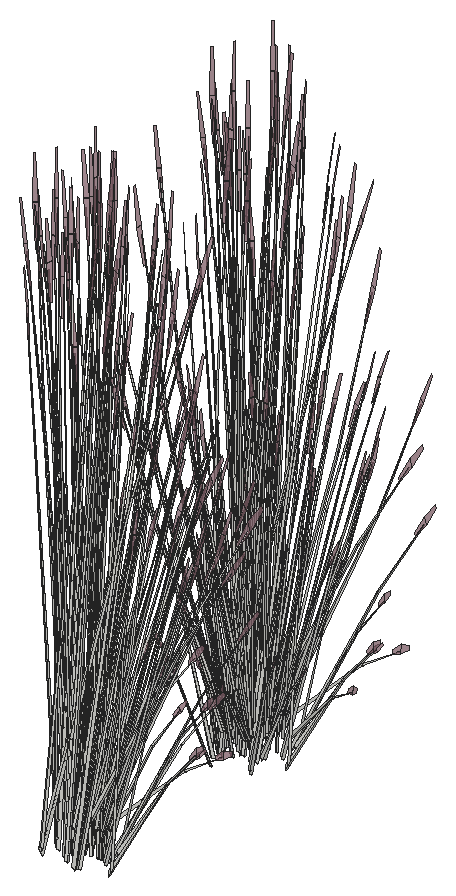
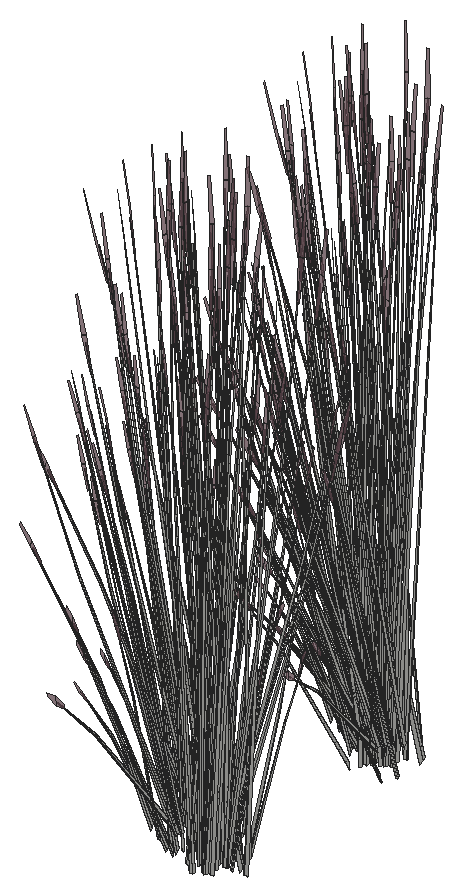
# SketchUp Ruby script. Lengths in inches.
U = 1.inch
M = Sketchup.active_model
def pt(a) = Geom::Point3d.new(a.map { |v| v * U })
def face(e, loops, mat)
  f = e.add_face(loops[0].map { |a| pt(a) })
  loops[1..].each { |l| e.add_face(l.map { |a| pt(a) }).erase! }
  f.material = f.back_material = mat if mat
  f
end
# faces: each face lists its corners as indices into pts; further lists are holes
def faces(e, pts, list, mat = nil) = list.each { |f| face(e, (f[0].is_a?(Array) ? f : [f]).map { |l| l.map { |i| pts[i] } }, mat) }
# xy, xz, yz: faces in a plane at the given z, y or x. An outline is a flat list of corners, or four numbers for a rectangle; further outlines are holes
def ring(l) = l.size == 4 ? [[l[0], l[1]], [l[2], l[1]], [l[2], l[3]], [l[0], l[3]]] : l.each_slice(2).to_a
def flat(e, list, mat, &to3) = list.each { |f| face(e, (f[0].is_a?(Array) ? f : [f]).map { |l| ring(l).map { |u, v| to3.(u, v) } }, mat) }
def xy(e, z, list, mat = nil) = flat(e, list, mat) { |x, y| [x, y, z] }
def xz(e, y, list, mat = nil) = flat(e, list, mat) { |x, z| [x, y, z] }
def yz(e, x, list, mat = nil) = flat(e, list, mat) { |y, z| [x, y, z] }
def lines(e, pts, list) = list.each { |a, b| e.add_line(pt(pts[a]), pt(pts[b])) }
# prism: a flat outline (further loops are holes) pulled along v
def prism(e, loops, v, mat = nil)
  f = face(e, loops, mat); d = Geom::Vector3d.new(v.map { |x| x * U })
  f.pushpull(f.normal.samedirection?(d) ? d.length : -d.length)
end
def box(e, o, s, mat = nil) = prism(e, [[o, [o[0] + s[0], o[1], o[2]], [o[0] + s[0], o[1] + s[1], o[2]], [o[0], o[1] + s[1], o[2]]]], [0, 0, s[2]], mat)
def at(x, y, z, deg = 0) = Geom::Transformation.translation(pt([x, y, z])) * Geom::Transformation.rotation(ORIGIN, Z_AXIS, deg.degrees)
def axes(o, x, y, z) = Geom::Transformation.new([*x, 0, *y, 0, *z, 0, *pt(o).to_a, 1])
def part(name) = M.definitions.add(name)
# library, detail: a bought-in or finely detailed component or shape, given as its bounding box
def library(name, o, s) = part(name).tap { |d| box(d.entities, o, s) }
def detail(e, o, s) = box(e.add_group.entities, o, s)
def put(e, d, t, mat = nil) = e.add_instance(d, t).tap { |i| i.material = mat if mat }
def group(e, t, mat = nil) = e.add_group.tap { |g| g.transformation = t; g.material = mat if mat }.entities
root = M.entities
M.materials.add("LightPink_Translucent").color = [144, 107, 117]
M.materials["LightPink_Translucent"].alpha = 0.75
c1 = part("blade")
p = [[2.15,0.21,22],[0,0.17,0],[0.09,0.45,0],[2.18,0.31,22],[2.29,0.31,22],[0.38,0.45,0],
  [2.48,0.24,33],[2.49,0.24,33],[2.48,0.22,33]]
faces(c1.entities,p,[[0,1,2,3],[4,5,2,3],[6,3,4,7],[8,0,3,6]])
c2 = part("seeds")
p = [[0.3,-0.1,1.38],[-0.01,-0.03,1.59],[-0.01,-0.03,0.03],[0.14,-0.07,-0.07],[0.29,-0.03,3],[0.15,0.01,3.11]]
faces(c2.entities,p,[[0,1,2,3],[1,0,4,5]],"LightPink_Translucent")
c3 = part("blade with seeds")
put(c3.entities,c1,at(0,0,0))
put(c3.entities,c2,axes([2.4,0.25,30.99],[1.5799,-0.05474,1.17369],[-0.12525,1.92788,0.29478],[-0.07173,-0.02425,1.56792]))
put(root,c3,axes([509.35,499.15,3.875],[0.20584,-0.55581,-0.51099],[0.70573,0.19051,-0.3958],[0.28414,-0.05097,0.97773]))
put(root,c3,axes([508.24,496.89,1.57],[0.47504,-0.61229,0],[0.79476,0.34146,-0.51607],[0.18101,0.07777,1.63711]))
put(root,c3,axes([505.49,498.78,1.55],[0.33034,0.68327,0.45755],[-0.94388,0.2376,0.17955],[0.01154,-0.12555,1.58856]))
put(root,c3,axes([510.11,499.31,1.17],[-0.48937,0.07333,1.41583],[-0.07789,-0.58369,0.08104],[0.34275,-0.08835,0.80566]))
put(root,c3,axes([511,498.79,1.45],[-0.47106,-0.39072,-0.06488],[0.51591,-0.35801,-0.29416],[0.14618,-0.02521,0.97024]))
put(root,c3,axes([505.32,499.32,1.91],[-0.36864,0.55059,0.44739],[-0.76598,-0.26498,-0.21531],[0,-0.12692,1.43643]))
put(root,c3,axes([506.67,498.84,1.4],[0,-0.70701,0],[0.95008,0,0],[0,0,1.79456]))
put(root,c3,axes([507.83,497.21,1.67],[-0.7111,-0.30552,0.49651],[0.42504,-0.54784,0],[0.16196,0.06958,1.57504]))
put(root,c3,axes([509.22,499.35,4.17],[0.66765,-0.26986,-0.71045],[0.37208,0.55551,0.08574],[0.32259,-0.0631,1.00501]))
put(root,c3,axes([506.22,498.39,1.55],[-0.62999,0.55453,0.45755],[-0.74845,-0.4895,0.17955],[0.15188,-0.05534,1.58856]))
put(root,c3,axes([506.91,499.39,1.49],[-0.70674,-0.52593,-0.06131],[0.70717,-0.52625,0],[-0.02468,-0.01837,1.75571]))
put(root,c3,axes([505.13,497.48,1.67],[-0.21949,0.60727,0.17642],[-0.8032,-0.17185,0.35086],[0.13875,-0.00296,1.60407]))
put(root,c3,axes([509.12,499.46,4.24],[-0.63144,-0.17046,0.35414],[0.18417,-0.49731,-0.4572],[0.25423,-0.0456,0.87481]))
put(root,c3,axes([504.8,497.97,0.79],[-0.74787,0.24464,1.28929],[-0.23804,-0.70192,0.50096],[0.45924,0.01168,1.46642]))
put(root,c3,axes([506.81,498.16,1.81],[0.14658,-0.54532,0.1448],[0.71613,0.09466,-0.41347],[0.13033,0.05599,1.26744]))
put(root,c3,axes([505.57,499.45,1.55],[0.96033,0.12874,0.45755],[-0.19544,0.7271,0.17955],[-0.14034,-0.07021,1.58856]))
put(root,c3,axes([510.64,498.92,0.6875],[-0.03971,-0.09277,1.76342],[0.27541,-0.54264,-0.26939],[0.27782,-0.00781,0.30037]))
put(root,c3,axes([506.5,498.3,1.91],[-0.45644,-0.51287,0.44739],[0.69137,-0.36116,-0.21531],[0.14771,0.06346,1.43643]))
put(root,c3,axes([505.05,500.61,1.67],[0.81646,-0.16218,0.17642],[0.20161,0.60355,0.35086],[-0.07282,-0.08794,1.60407]))
put(root,c3,axes([506.73,498.33,1.86],[0.76714,-0.40567,-0.29095],[0.51013,0.57321,-0.50002],[0.18927,0.05821,1.59708]))
put(root,c3,axes([509.78,499.4,3.72],[0.63144,0.17046,-0.35414],[-0.18417,0.49731,0.4572],[0.25423,-0.0456,0.87481]))
put(root,c3,axes([508.67,497.26,1.21],[0.7111,0.30552,-0.49651],[-0.42504,0.54784,0],[0.16196,0.06958,1.57504]))
put(root,c3,axes([507.32,499,1.4],[0.85008,0,0],[0,0.63259,0],[0,0,1.78407]))
put(root,c3,axes([507.56,497.51,1.67],[-0.81646,0.16218,0.17642],[-0.20161,-0.60355,0.35086],[0.07282,0.08794,1.60407]))
put(root,c3,axes([508.0625,498.79,3.07],[-0.31515,0.01384,1.71376],[0.20907,-0.5998,0.13857],[0.44912,0.0371,0.73262]))
put(root,c3,axes([508.47,497.48,1.22],[0.17848,0.53243,-0.30978],[-0.70886,0.15119,0.30978],[0.1429,0.0614,1.38974]))
put(root,c3,axes([509.69,499.61,3.92],[0.27906,0.41663,0.0643],[-0.50888,0.20393,0.50621],[0.22432,-0.04024,0.77189]))
put(root,c3,axes([507.04,498.68,1.57],[-0.96033,-0.12874,0.49198],[0.19544,-0.7271,0.19306],[0.14034,0.07021,1.70813]))
put(root,c3,axes([509.64,499.46,3.93],[-0.21466,0.55714,0.48003],[-0.70573,-0.19051,0.3958],[0.27753,-0.03348,0.9933]))
put(root,c3,axes([506.28,500.47,1.4],[-0.24791,-0.5268,0],[0.70791,-0.18448,0],[0,0,1.54371]))
put(root,c3,axes([507.21,500.4,1.38],[0.79769,-0.20732,-0.19198],[0.2803,0.59721,0.00008],[0.08805,-0.02292,1.73897]))
put(root,c3,axes([507.48,500.65,1.67],[0.21949,-0.60727,0.17642],[0.8032,0.17185,0.35086],[-0.13875,0.00296,1.60407]))
put(root,c3,axes([507.3,499.27,1.41],[0.53038,0.39469,0],[-0.53038,0.39469,0],[0,0,1.69266]))
put(root,c3,axes([508.74,499.1,1.67],[-0.59697,-0.44509,0.17642],[0.60159,-0.4317,0.35086],[-0.06593,0.0909,1.60407]))
put(root,c3,axes([507.63,498.43,1.25],[0.79037,0.10018,-0.62353],[-0.16679,0.61794,-0.16365],[0.23587,0.07488,1.37633]))
put(root,c3,axes([511.125,499.5,1.96],[-0.46945,0.10088,1.1486],[0.22097,-0.4169,0.84392],[0.24904,0.02853,0.25299]))
put(root,c3,axes([506.1,500.71,1.39],[-0.76598,-0.27433,0],[0.36864,-0.57001,0],[0,0,1.62707]))
put(root,c3,axes([507.29,498.81,1.91],[0.36864,-0.55059,0.44739],[0.76598,0.26498,-0.21531],[0,0.12692,1.43643]))
put(root,c3,axes([510.91,501.27,3.9],[-0.0687,-0.05349,1.77383],[0.15029,-0.57341,-0.16761],[0.27062,-0.03664,0.31391]))
put(root,c3,axes([507.15,499.12,1.48],[0,0.70667,-0.05637],[-0.95008,0,0],[0,0.02221,1.79368]))
put(root,c3,axes([507.22,498.62,1.4],[0.45644,0.51287,-0.44739],[-0.69137,0.36116,0.21531],[0.14771,0.06346,1.43643]))
put(root,c3,axes([510.31,500.79,3.12],[-0.14542,-0.51365,-0.03492],[0.68734,-0.11809,-0.15832],[0.14353,0.03256,0.52218]))
put(root,c3,axes([508.53,500.77,4.23],[0.04068,-0.62141,-0.1216],[0.77029,0.01698,-0.67495],[0.29667,0.04317,1.02557]))
put(root,c3,axes([509.23,499.11,1.67],[0,-0.61104,0.49651],[0.85008,0,0],[0,0.13917,1.57504]))
put(root,c3,axes([507.1,499.57,1.91],[0.82508,-0.03772,0.44739],[0.07462,0.62614,-0.21531],[-0.14771,0.06346,1.43643]))
put(root,c3,axes([507.61,498.93,1.81],[0.70791,-0.1782,0.1448],[0.24791,0.50885,-0.41347],[0,0.11199,1.26744]))
put(root,c3,axes([508.41,500.53,4.24],[-0.43232,-0.38257,0.35414],[0.49364,-0.36215,-0.4572],[0.25081,0.0551,0.87481]))
put(root,c3,axes([510.24,500.17,1.78],[-0.18299,-0.15028,1.43002],[0.23809,-0.49714,-0.30754],[0.37023,0.06735,0.61141]))
put(root,c3,axes([506.97,500.72,1.4],[0.76598,0.27433,0],[-0.36864,0.57001,0],[0,0,1.74954]))
put(root,c3,axes([509.2,500.4,3.91],[0.16299,-0.01033,1.74944],[0.44707,-0.47471,-0.27667],[0.28992,0.06266,0.14031]))
put(root,c3,axes([507.11,499.84,1.81],[0.56134,0.36712,0.1448],[-0.46823,0.41419,-0.41347],[-0.13033,0.05599,1.26744]))
put(root,c3,axes([508.5625,500.48,4.17],[0.75952,0.01471,-0.71045],[-0.05101,0.61953,0.08574],[0.32177,0.06538,1.00501]))
put(root,c3,axes([507.71,500.97,1.67],[0.7111,-0.30552,0.49651],[0.42504,0.54784,0],[-0.16196,0.06958,1.57504]))
put(root,c3,axes([506.7,500.49,1.48],[0.33034,0.70197,-0.06012],[-0.94388,0.24598,0],[0.01154,0.02451,1.72173]))
put(root,c3,axes([509.81,499.22,1.57],[0.95008,0,0],[0,0.68292,-0.51607],[0,0.15554,1.63711]))
put(root,c3,axes([509.43,499.57,1.39],[-0.94962,-0.00489,-0.04976],[0,-0.68292,0.49943],[-0.02984,0.15546,1.58352]))
put(root,c3,axes([507.37,498.97,1.86],[0.85568,0.29155,-0.29095],[-0.41201,0.61537,-0.50002],[0.02689,0.15109,1.59708]))
put(root,c3,axes([509.02,500.73,3.72],[0.43232,0.38257,-0.35414],[-0.49364,0.36215,0.4572],[0.25081,0.0551,0.87481]))
put(root,c3,axes([509.23,499.67,1.22],[-0.53038,0.38124,-0.30978],[-0.53038,-0.38124,0.30978],[0,0.1228,1.38974]))
put(root,c3,axes([506.94,499.71,1.86],[0.08854,0.69723,-0.29095],[-0.92215,0.04216,-0.50002],[-0.16238,0.09287,1.59708]))
put(root,c3,axes([508.8,500.88,3.92],[-0.03826,0.46465,0.0643],[-0.57772,-0.01274,0.50621],[0.2213,0.04862,0.77189]))
put(root,c3,axes([507.28,499.43,1.4],[-0.36864,0.55059,-0.44739],[-0.76598,-0.26498,0.21531],[0,0.12692,1.43643]))
put(root,c3,axes([508.85,500.73,3.93],[-0.56024,0.40262,0.48003],[-0.48318,-0.42758,0.3958],[0.26285,0.07427,0.9933]))
put(root,c3,axes([507.07,501.2,4.24],[-0.11735,-0.49217,0.35414],[0.67083,-0.12996,-0.4572],[0.18018,0.14104,0.87481]))
put(root,c3,axes([507.3,501.01,1.52],[0.95122,0.19861,0.30756],[-0.23797,0.7099,-0.36492],[-0.15744,0.08885,1.64885]))
put(root,c3,axes([509.59,499.68,1.21],[0,0.61104,-0.49651],[-0.85008,0,0],[0,0.13917,1.57504]))
put(root,c3,axes([507.47,499.75,3.07],[-0.28223,-0.10528,1.71376],[0.58406,-0.44165,0.13857],[0.36402,0.19924,0.73262]))
put(root,c3,axes([507.52,498.36,3.67],[-0.65655,-0.31748,1.38283],[0.69326,-0.49431,0.59665],[0.21183,0.29789,1.33663]))
put(root,c3,axes([508.51,500.95,1.96],[-0.4278,-0.1757,1.1486],[0.5524,-0.17852,0.84392],[0.14899,0.15122,0.25299]))
put(root,c3,axes([507.01,501.45,4.23],[0.45276,-0.52302,-0.1216],[0.65568,0.30132,-0.67495],[0.22792,0.14777,1.02557]))
put(root,c3,axes([504.03,500.74,4.24],[0.5141,-0.32171,0.35414],[0.48666,0.36734,-0.4572],[-0.07405,0.18664,0.87481]))
put(root,c3,axes([507.875,501.4,1.57],[0.47504,0.61229,0],[-0.79476,0.34146,-0.51607],[-0.18101,0.07777,1.63711]))
put(root,c3,axes([506.42,501.88,3.9],[0.00225,-0.07398,1.77383],[0.65113,-0.32638,-0.16761],[0.22617,0.1165,0.31391]))
put(root,c3,axes([508.63,501.6,0.6875],[0.05536,-0.08822,1.76342],[0.69692,-0.25981,-0.26939],[0.21129,0.13447,0.30037]))
put(root,c3,axes([507.47,498.97,2.03],[-0.02076,-0.57531,1.41272],[0.93937,0.14913,0.59816],[-0.22217,0.31481,1.3335]))
put(root,c3,axes([507.71,499.6,1.29],[0.2786,0.55945,-0.69212],[-0.80253,0.20149,-0.18165],[0.03079,0.18945,1.52773]))
put(root,c3,axes([507.55,501.19,3.875],[0.74975,-0.14525,-0.51099],[0.13115,0.55007,-0.3958],[0.20138,0.15763,0.97773]))
put(root,c3,axes([505.47,501.27,4.24],[0.22906,-0.4699,0.35414],[0.66828,0.13705,-0.4572],[0.06128,0.18919,0.87481]))
put(root,c3,axes([508.58,501.75,1.86],[-0.48723,-0.01916,1.0506],[0.32177,-0.40701,0.58006],[0.19248,0.1446,0.8241]))
put(root,c3,axes([507.18,501.64,3.92],[-0.34533,0.38816,0.0643],[-0.49176,-0.22599,0.50621],[0.15898,0.12445,0.77189]))
put(root,c3,axes([506.37,502.95,4.84],[0.52505,-0.35054,-0.06488],[0.48109,0.38392,-0.29416],[0.03387,0.10878,0.97024]))
put(root,c3,axes([507.32,501.53,3.93],[-0.75571,0.14023,0.48003],[-0.13115,-0.55007,0.3958],[0.17773,0.16212,0.9933]))
put(root,c3,axes([506.99,500.76,1.78],[0.01341,-0.20255,1.43002],[0.64074,-0.22625,-0.30754],[0.1978,0.24243,0.61141]))
put(root,c3,axes([505.26,501.7,3.92],[-0.55987,0.20767,0.0643],[-0.27403,-0.37869,0.50621],[0.05407,0.16693,0.77189]))
put(root,c3,axes([503.7,500.83,4.59],[0.83505,0.03027,-0.13498],[-0.02282,0.57322,-0.74919],[-0.05801,0.22077,1.13838]))
put(root,c3,axes([505.24,501.47,4.23],[0.74352,-0.28449,-0.1216],[0.36538,0.50492,-0.67495],[0.0981,0.21277,1.02557]))
put(root,c3,axes([505.46,501.66,4.26],[-0.74868,-0.15974,0.53283],[0.25601,-0.52518,0.43934],[0.04499,0.20653,1.10256]))
put(root,c3,axes([505.38,501.58,0.6875],[0.12297,-0.03325,1.76342],[0.73967,0.18301,-0.26939],[0.02163,0.20626,0.30037]))
put(root,c3,axes([503.68,501.67,2.02],[0.69024,-0.1082,0.06507],[0.15868,0.43593,-0.86304],[-0.04376,0.22067,0.7736]))
put(root,c3,axes([505.88,501.45,3.875],[0.7469,0.15318,-0.51099],[-0.25601,0.52518,-0.3958],[0.06849,0.21144,0.97773]))
put(root,c3,axes([506.31,500.36,3.07],[-0.17368,-0.19618,1.71376],[0.80256,-0.16516,0.13857],[0.18139,0.30799,0.73262]))
put(root,c3,axes([505.54,501.77,3.72],[-0.22906,0.4699,-0.35414],[-0.66828,-0.13705,0.4572],[0.06128,0.18919,0.87481]))
put(root,c3,axes([504.89,500.46,3.07],[-0.0186,-0.23452,1.71376],[0.80601,0.15558,0.13857],[-0.04985,0.33422,0.73262]))
put(root,c3,axes([505.61,501.35,4.17],[0.36264,0.49684,-0.71045],[-0.74649,0.27689,0.08574],[0.0848,0.24006,1.00501]))
put(root,c3,axes([505.07,502.6,3.91],[0.09631,0.0984,1.74944],[0.77725,0.03866,-0.27667],[0.07816,0.217,0.14031]))
put(root,c3,axes([507.76,518.33,1.78],[-0.21597,0.12368,1.43002],[-0.64681,-0.21647,-0.30754],[0.1199,-0.26922,0.61141]))
put(root,c3,axes([506.77,518.77,4.17],[-0.36264,-0.49684,-0.71045],[0.74649,-0.27689,0.08574],[-0.0848,-0.24006,1.00501]))
put(root,c3,axes([506.15,517.66,0.6875],[-0.12744,0.02202,1.76342],[-0.70477,-0.24781,-0.26939],[0.01183,-0.2067,0.30037]))
put(root,c3,axes([508.28,519.25,4.17],[0.01977,-0.56521,-0.71045],[0.83252,0.03796,0.08574],[0.08786,-0.23945,1.00501]))
put(root,c3,axes([509.44,518.37,3.91],[-0.00733,-0.12161,1.74944],[-0.61946,-0.35147,-0.27667],[0.09577,-0.21306,0.14031]))
put(root,c3,axes([506.84,518.34,3.72],[0.22906,-0.4699,-0.35414],[0.66828,0.13705,0.4572],[-0.06128,-0.18919,0.87481]))
put(root,c3,axes([507.34,518.96,3.07],[-0.14147,0.21002,1.71376],[-0.59349,-0.43464,0.13857],[0.26773,-0.27089,0.73262]))
put(root,c3,axes([509.28,517.93,3.9],[-0.07716,0.04667,1.77383],[-0.75601,-0.15746,-0.16761],[-0.02737,-0.20368,0.31391]))
put(root,c3,axes([506.5,518.67,3.875],[-0.7469,-0.15318,-0.51099],[0.25601,-0.52518,-0.3958],[-0.06849,-0.21144,0.97773]))
put(root,c3,axes([506.96,517.35,1.96],[0.09747,0.35631,1.1486],[-0.54071,-0.19735,0.84392],[0.05818,-0.18244,0.25299]))
put(root,c3,axes([508.11,519.0625,3.875],[-0.54391,-0.41056,-0.51099],[0.57458,-0.35956,-0.3958],[0.08276,-0.2086,0.97773]))
put(root,c3,axes([506.92,518.45,3.93],[0.74868,0.15974,0.48003],[-0.25601,0.52518,0.3958],[-0.04499,-0.20653,0.9933]))
put(root,c3,axes([507.14,518.64,4.23],[-0.74352,0.28449,-0.1216],[-0.36538,-0.50492,-0.67495],[-0.0981,-0.21277,1.02557]))
put(root,c3,axes([508.68,519.28,4.23],[-0.83505,-0.03027,-0.1216],[0.02282,-0.57322,-0.67495],[0.05801,-0.22077,1.02557]))
put(root,c3,axes([508.625,518.91,3.72],[0.5141,-0.32171,-0.35414],[0.48666,0.36734,0.4572],[0.07405,-0.18664,0.87481]))
put(root,c3,axes([507.12,518.41,3.92],[0.55987,-0.20767,0.0643],[0.27403,0.37869,0.50621],[-0.05407,-0.16693,0.77189]))
put(root,c3,axes([505.09,520.63,1.29],[-0.31203,-0.62659,-0.69835],[0.89884,-0.22566,-0.18329],[-0.03449,-0.21218,1.54149]))
put(root,c3,axes([509.27,518.72,0.6875],[-0.11372,-0.04814,1.76342],[-0.29211,-0.53779,-0.26939],[0.19706,-0.14594,0.30037]))
put(root,c3,axes([506.91,518.84,4.24],[-0.22906,0.4699,0.35414],[-0.66828,-0.13705,-0.4572],[-0.06128,-0.18919,0.87481]))
put(root,c3,axes([508.62,519.04,3.93],[0.54105,0.41691,0.48003],[-0.57458,0.35956,0.3958],[0.0998,-0.1956,0.9933]))
put(root,c3,axes([508.82,519.08,3.92],[0.62439,0.02847,0.0643],[-0.01712,0.42991,0.50621],[0.06534,-0.16468,0.77189]))
put(root,c3,axes([508.36,519.37,4.24],[-0.5141,0.32171,0.35414],[-0.48666,-0.36734,-0.4572],[0.07405,-0.18664,0.87481]))
put(root,c3,axes([509.26,520.23,4.17],[0.39688,-0.48213,-0.71045],[0.69548,0.34264,0.08574],[0.23697,-0.17468,1.00501]))
put(root,c3,axes([504.97,518.83,1.57],[-0.47504,-0.61229,0],[0.79476,-0.34146,-0.51607],[0.18101,-0.07777,1.63711]))
put(root,c3,axes([509.24,520.01,3.875],[-0.19519,-0.55794,-0.51099],[0.73919,-0.0976,-0.3958],[0.21183,-0.14986,0.97773]))
put(root,c3,axes([506.01,518.09,1.32],[-0.52505,0.35054,-0.03893],[-0.48109,-0.38392,-0.17649],[-0.03387,-0.10878,0.58215]))
put(root,c3,axes([509.59,520.41,4.23],[-0.70283,-0.33692,-0.1216],[0.40491,-0.48793,-0.67495],[0.19857,-0.16961,1.02557]))
put(root,c3,axes([505.62,518.73,1.21],[0.7111,-0.30552,-0.49651],[0.42504,0.54784,0],[0.16196,-0.06958,1.57504]))
put(root,c3,axes([509.84,519.79,1.78],[-0.27143,-0.0181,1.43002],[-0.27808,-0.48551,-0.30754],[0.33346,-0.13735,0.61141]))
put(root,c3,axes([511.32,520.26,3.9],[-0.09924,-0.00464,1.77383],[-0.4121,-0.49725,-0.16761],[0.1655,-0.1635,0.31391]))
put(root,c3,axes([506.46,519.99,1.25],[0.51177,-0.45928,-0.62353],[0.63575,0.41646,-0.16365],[0.20507,-0.11457,1.37633]))
put(root,c3,axes([510.15,518.9,1.96],[-0.25308,0.31105,1.1486],[-0.21753,-0.4179,0.84392],[0.20902,-0.10472,0.25299]))
put(root,c3,axes([509.79,520.07,3.72],[0.66138,-0.08733,-0.35414],[0.17464,0.49921,0.4572],[0.18953,-0.13408,0.87481]))
put(root,c3,axes([505.57,520.79,1.4],[0.36864,-0.55059,-0.44739],[0.76598,0.26498,0.21531],[0,-0.12692,1.43643]))
put(root,c3,axes([505.9,520.52,1.86],[-0.08854,-0.69723,-0.29095],[0.92215,-0.04216,-0.50002],[0.16238,-0.09287,1.59708]))
put(root,c3,axes([503.62,520.56,1.22],[0.53038,-0.38124,-0.30978],[0.53038,0.38124,0.30978],[0,-0.1228,1.38974]))
put(root,c3,axes([509.25,520.36,4.24],[-0.66138,0.08733,0.35414],[-0.17464,-0.49921,-0.4572],[0.18953,-0.13408,0.87481]))
put(root,c3,axes([505.48,521.25,1.86],[-0.85568,-0.29155,-0.29095],[0.41201,-0.61537,-0.50002],[-0.02689,-0.15109,1.59708]))
put(root,c3,axes([505.78,518.98,1.22],[0.70886,0.15119,-0.30978],[-0.17848,0.53243,0.30978],[0.1429,-0.0614,1.38974]))
put(root,c3,axes([509.85,520.28,3.92],[0.52161,0.25698,0.0643],[-0.30368,0.36595,0.50621],[0.16723,-0.11831,0.77189]))
put(root,c3,axes([509.7,520.17,3.93],[0.18844,0.56237,0.48003],[-0.73919,0.0976,0.3958],[0.21785,-0.13226,0.9933]))
put(root,c3,axes([511.7,520.86,3.91],[0.10543,-0.09307,1.74944],[-0.13495,-0.57092,-0.27667],[0.26455,-0.10825,0.14031]))
put(root,c3,axes([506.03,521.07,1.625],[0.8561,0.29616,0.24065],[-0.41201,0.61537,0.50002],[0,-0.14185,1.60543]))
put(root,c3,axes([505.75,520.65,1.91],[-0.82508,0.03772,0.44739],[-0.07462,-0.62614,-0.21531],[0.14771,-0.06346,1.43643]))
put(root,c3,axes([509.62,521.72,4.23],[-0.38229,-0.5533,-0.1216],[0.6785,-0.2719,-0.67495],[0.28593,-0.073,1.02557]))
put(root,c3,axes([509.59,521.25,3.875],[0.20584,-0.55581,-0.51099],[0.70573,0.19051,-0.3958],[0.28414,-0.05097,0.97773]))
put(root,c3,axes([508.47,518.98,1.57],[0.47504,-0.61229,0],[0.79476,0.34146,-0.51607],[0.18101,0.07777,1.63711]))
put(root,c3,axes([505.72,520.88,1.55],[0.33034,0.68327,0.45755],[-0.94388,0.2376,0.17955],[0.01154,-0.12555,1.58856]))
put(root,c3,axes([510.34,521.4,1.17],[-0.48937,0.07333,1.41583],[-0.07789,-0.58369,0.08104],[0.34275,-0.08835,0.80566]))
put(root,c3,axes([511.23,520.89,1.45],[-0.47106,-0.39072,-0.06488],[0.51591,-0.35801,-0.29416],[0.14618,-0.02521,0.97024]))
put(root,c3,axes([505.55,521.42,1.91],[-0.36864,0.55059,0.44739],[-0.76598,-0.26498,-0.21531],[0,-0.12692,1.43643]))
put(root,c3,axes([506.91,520.9375,1.4],[0,-0.70701,0],[0.95008,0,0],[0,0,1.79456]))
put(root,c3,axes([508.06,519.3,1.67],[-0.7111,-0.30552,0.49651],[0.42504,-0.54784,0],[0.16196,0.06958,1.57504]))
put(root,c3,axes([509.45,521.45,4.17],[0.66765,-0.26986,-0.71045],[0.37208,0.55551,0.08574],[0.32259,-0.0631,1.00501]))
put(root,c3,axes([506.46,520.49,1.55],[-0.62999,0.55453,0.45755],[-0.74845,-0.4895,0.17955],[0.15188,-0.05534,1.58856]))
put(root,c3,axes([507.15,521.49,1.49],[-0.70674,-0.52593,-0.06131],[0.70717,-0.52625,0],[-0.02468,-0.01837,1.75571]))
put(root,c3,axes([505.36,519.58,1.67],[-0.21949,0.60727,0.17642],[-0.8032,-0.17185,0.35086],[0.13875,-0.00296,1.60407]))
put(root,c3,axes([509.35,521.56,4.24],[-0.63144,-0.17046,0.35414],[0.18417,-0.49731,-0.4572],[0.25423,-0.0456,0.87481]))
put(root,c3,axes([505.03,520.07,0.79],[-0.74787,0.24464,1.28929],[-0.23804,-0.70192,0.50096],[0.45924,0.01168,1.46642]))
put(root,c3,axes([507.04,520.25,1.81],[0.14658,-0.54532,0.1448],[0.71613,0.09466,-0.41347],[0.13033,0.05599,1.26744]))
put(root,c3,axes([505.8,521.55,1.55],[0.96033,0.12874,0.45755],[-0.19544,0.7271,0.17955],[-0.14034,-0.07021,1.58856]))
put(root,c3,axes([510.875,521.02,0.6875],[-0.03971,-0.09277,1.76342],[0.27541,-0.54264,-0.26939],[0.27782,-0.00781,0.30037]))
put(root,c3,axes([506.74,520.4,1.91],[-0.45644,-0.51287,0.44739],[0.69137,-0.36116,-0.21531],[0.14771,0.06346,1.43643]))
put(root,c3,axes([505.29,522.71,1.67],[0.81646,-0.16218,0.17642],[0.20161,0.60355,0.35086],[-0.07282,-0.08794,1.60407]))
put(root,c3,axes([506.97,520.43,1.86],[0.76714,-0.40567,-0.29095],[0.51013,0.57321,-0.50002],[0.18927,0.05821,1.59708]))
put(root,c3,axes([510.02,521.5,3.72],[0.63144,0.17046,-0.35414],[-0.18417,0.49731,0.4572],[0.25423,-0.0456,0.87481]))
put(root,c3,axes([508.9,519.35,1.21],[0.7111,0.30552,-0.49651],[-0.42504,0.54784,0],[0.16196,0.06958,1.57504]))
put(root,c3,axes([507.55,521.1,1.4],[0.85008,0,0],[0,0.63259,0],[0,0,1.78407]))
put(root,c3,axes([507.79,519.61,1.67],[-0.81646,0.16218,0.17642],[-0.20161,-0.60355,0.35086],[0.07282,0.08794,1.60407]))
put(root,c3,axes([508.3,520.89,3.07],[-0.31515,0.01384,1.71376],[0.20907,-0.5998,0.13857],[0.44912,0.0371,0.73262]))
put(root,c3,axes([508.7,519.58,1.22],[0.17848,0.53243,-0.30978],[-0.70886,0.15119,0.30978],[0.1429,0.0614,1.38974]))
put(root,c3,axes([509.93,521.71,3.92],[0.27906,0.41663,0.0643],[-0.50888,0.20393,0.50621],[0.22432,-0.04024,0.77189]))
put(root,c3,axes([507.28,520.77,1.57],[-0.96033,-0.12874,0.49198],[0.19544,-0.7271,0.19306],[0.14034,0.07021,1.70813]))
put(root,c3,axes([509.87,521.5625,3.93],[-0.21466,0.55714,0.48003],[-0.70573,-0.19051,0.3958],[0.27753,-0.03348,0.9933]))
put(root,c3,axes([506.51,522.57,1.4],[-0.24791,-0.5268,0],[0.70791,-0.18448,0],[0,0,1.54371]))
put(root,c3,axes([507.44,522.49,1.38],[0.79769,-0.20732,-0.19198],[0.2803,0.59721,0.00008],[0.08805,-0.02292,1.73897]))
put(root,c3,axes([507.72,522.74,1.67],[0.21949,-0.60727,0.17642],[0.8032,0.17185,0.35086],[-0.13875,0.00296,1.60407]))
put(root,c3,axes([507.53,521.37,1.41],[0.53038,0.39469,0],[-0.53038,0.39469,0],[0,0,1.69266]))
put(root,c3,axes([508.97,521.19,1.67],[-0.59697,-0.44509,0.17642],[0.60159,-0.4317,0.35086],[-0.06593,0.0909,1.60407]))
put(root,c3,axes([507.87,520.52,1.25],[0.79037,0.10018,-0.62353],[-0.16679,0.61794,-0.16365],[0.23587,0.07488,1.37633]))
put(root,c3,axes([511.36,521.6,1.96],[-0.46945,0.10088,1.1486],[0.22097,-0.4169,0.84392],[0.24904,0.02853,0.25299]))
put(root,c3,axes([506.34,522.81,1.39],[-0.76598,-0.27433,0],[0.36864,-0.57001,0],[0,0,1.62707]))
put(root,c3,axes([507.53,520.91,1.91],[0.36864,-0.55059,0.44739],[0.76598,0.26498,-0.21531],[0,0.12692,1.43643]))
put(root,c3,axes([511.14,523.37,3.9],[-0.0687,-0.05349,1.77383],[0.15029,-0.57341,-0.16761],[0.27062,-0.03664,0.31391]))
put(root,c3,axes([507.39,521.22,1.48],[0,0.70667,-0.05637],[-0.95008,0,0],[0,0.02221,1.79368]))
put(root,c3,axes([507.46,520.72,1.4],[0.45644,0.51287,-0.44739],[-0.69137,0.36116,0.21531],[0.14771,0.06346,1.43643]))
put(root,c3,axes([510.54,522.89,3.12],[-0.14542,-0.51365,-0.03492],[0.68734,-0.11809,-0.15832],[0.14353,0.03256,0.52218]))
put(root,c3,axes([508.76,522.87,4.23],[0.04068,-0.62141,-0.1216],[0.77029,0.01698,-0.67495],[0.29667,0.04317,1.02557]))
put(root,c3,axes([509.46,521.21,1.67],[0,-0.61104,0.49651],[0.85008,0,0],[0,0.13917,1.57504]))
put(root,c3,axes([507.33,521.67,1.91],[0.82508,-0.03772,0.44739],[0.07462,0.62614,-0.21531],[-0.14771,0.06346,1.43643]))
put(root,c3,axes([507.85,521.03,1.81],[0.70791,-0.1782,0.1448],[0.24791,0.50885,-0.41347],[0,0.11199,1.26744]))
put(root,c3,axes([508.64,522.63,4.24],[-0.43232,-0.38257,0.35414],[0.49364,-0.36215,-0.4572],[0.25081,0.0551,0.87481]))
put(root,c3,axes([510.48,522.27,1.78],[-0.18299,-0.15028,1.43002],[0.23809,-0.49714,-0.30754],[0.37023,0.06735,0.61141]))
put(root,c3,axes([507.21,522.82,1.4],[0.76598,0.27433,0],[-0.36864,0.57001,0],[0,0,1.74954]))
put(root,c3,axes([509.43,522.5,3.91],[0.16299,-0.01033,1.74944],[0.44707,-0.47471,-0.27667],[0.28992,0.06266,0.14031]))
put(root,c3,axes([507.35,521.9375,1.81],[0.56134,0.36712,0.1448],[-0.46823,0.41419,-0.41347],[-0.13033,0.05599,1.26744]))
put(root,c3,axes([508.8,522.57,4.17],[0.75952,0.01471,-0.71045],[-0.05101,0.61953,0.08574],[0.32177,0.06538,1.00501]))
